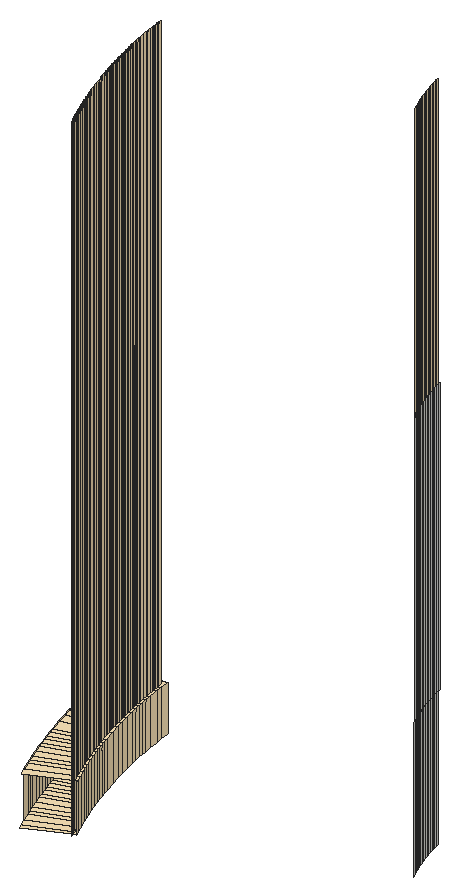
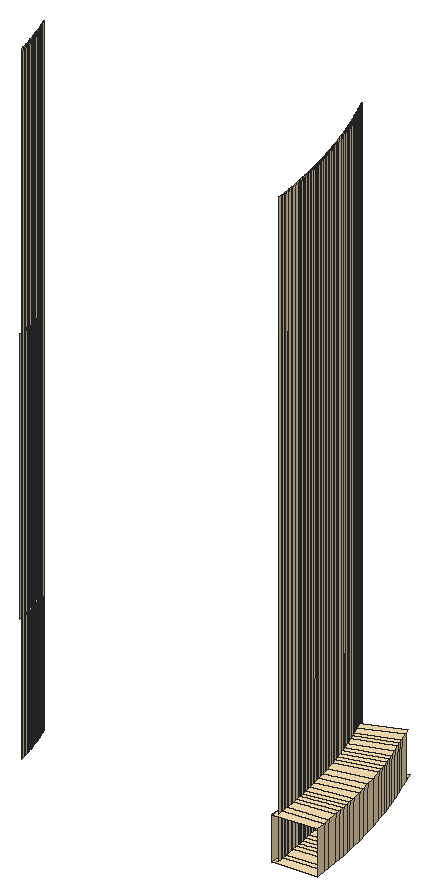
# SketchUp Ruby script. Lengths in inches.
U = 1.inch
M = Sketchup.active_model
def pt(a) = Geom::Point3d.new(a.map { |v| v * U })
def face(e, loops, mat)
  f = e.add_face(loops[0].map { |a| pt(a) })
  loops[1..].each { |l| e.add_face(l.map { |a| pt(a) }).erase! }
  f.material = f.back_material = mat if mat
  f
end
# faces: each face lists its corners as indices into pts; further lists are holes
def faces(e, pts, list, mat = nil) = list.each { |f| face(e, (f[0].is_a?(Array) ? f : [f]).map { |l| l.map { |i| pts[i] } }, mat) }
# xy, xz, yz: faces in a plane at the given z, y or x. An outline is a flat list of corners, or four numbers for a rectangle; further outlines are holes
def ring(l) = l.size == 4 ? [[l[0], l[1]], [l[2], l[1]], [l[2], l[3]], [l[0], l[3]]] : l.each_slice(2).to_a
def flat(e, list, mat, &to3) = list.each { |f| face(e, (f[0].is_a?(Array) ? f : [f]).map { |l| ring(l).map { |u, v| to3.(u, v) } }, mat) }
def xy(e, z, list, mat = nil) = flat(e, list, mat) { |x, y| [x, y, z] }
def xz(e, y, list, mat = nil) = flat(e, list, mat) { |x, z| [x, y, z] }
def yz(e, x, list, mat = nil) = flat(e, list, mat) { |y, z| [x, y, z] }
def lines(e, pts, list) = list.each { |a, b| e.add_line(pt(pts[a]), pt(pts[b])) }
# prism: a flat outline (further loops are holes) pulled along v
def prism(e, loops, v, mat = nil)
  f = face(e, loops, mat); d = Geom::Vector3d.new(v.map { |x| x * U })
  f.pushpull(f.normal.samedirection?(d) ? d.length : -d.length)
end
def box(e, o, s, mat = nil) = prism(e, [[o, [o[0] + s[0], o[1], o[2]], [o[0] + s[0], o[1] + s[1], o[2]], [o[0], o[1] + s[1], o[2]]]], [0, 0, s[2]], mat)
def at(x, y, z, deg = 0) = Geom::Transformation.translation(pt([x, y, z])) * Geom::Transformation.rotation(ORIGIN, Z_AXIS, deg.degrees)
def axes(o, x, y, z) = Geom::Transformation.new([*x, 0, *y, 0, *z, 0, *pt(o).to_a, 1])
def part(name) = M.definitions.add(name)
# library, detail: a bought-in or finely detailed component or shape, given as its bounding box
def library(name, o, s) = part(name).tap { |d| box(d.entities, o, s) }
def detail(e, o, s) = box(e.add_group.entities, o, s)
def put(e, d, t, mat = nil) = e.add_instance(d, t).tap { |i| i.material = mat if mat }
def group(e, t, mat = nil) = e.add_group.tap { |g| g.transformation = t; g.material = mat if mat }.entities
root = M.entities
M.materials.add("1026 AP 7946 SUNNY SIDE UP").color = [254, 231, 186]
xy(root,246,[[6.415,228.386,6.327,228.585,8.035,229.33,8.046,229.304,8.075,229.238,8.09,229.204,8.107,229.167,8.114,229.152],[6.327,228.585,6.202,228.876,7.918,229.598,7.948,229.528,7.974,229.468,7.992,229.428,8.011,229.382,8.035,229.33],[6.202,228.876,6.034,229.281,7.76,229.98,7.779,229.932,7.802,229.878,7.827,229.816,7.853,229.754,7.875,229.7,7.896,229.652,7.918,229.598],[8.114,229.152,8.107,229.167,8.09,229.204,8.075,229.238,8.046,229.304,8.035,229.33,8.16,229.384,8.238,229.208],[6.034,229.281,5.939,229.52,7.672,230.199,7.685,230.165,7.71,230.104,7.738,230.034,7.76,229.98],
  [8.035,229.33,8.011,229.382,7.992,229.428,7.974,229.468,7.948,229.528,7.918,229.598,8.045,229.652,8.16,229.384],[5.939,229.52,5.847,229.76,7.587,230.418,7.594,230.399,7.62,230.333,7.651,230.253,7.669,230.207,7.672,230.199],[7.918,229.598,7.896,229.652,7.875,229.7,7.853,229.754,7.827,229.816,7.802,229.878,7.779,229.932,7.76,229.98,7.888,230.032,8.045,229.652],[5.847,229.76,5.719,230.103,7.467,230.739,7.483,230.693,7.495,230.662,7.505,230.634,7.532,230.5625,7.566,230.473,7.581,230.434,7.587,230.418],[7.76,229.98,7.738,230.034,7.71,230.104,7.685,230.165,7.672,230.199,7.802,230.249,7.888,230.032],
  [5.719,230.103,5.6,230.438,7.355,231.052,7.362,231.03,7.403,230.915,7.411,230.892,7.419,230.87,7.447,230.794,7.467,230.739],[7.672,230.199,7.669,230.207,7.651,230.253,7.62,230.333,7.594,230.399,7.587,230.418,7.718,230.467,7.802,230.249],[7.587,230.418,7.581,230.434,7.566,230.473,7.532,230.5625,7.505,230.634,7.495,230.662,7.483,230.693,7.467,230.739,7.599,230.787,7.718,230.467],[5.6,230.438,5.512,230.696,7.273,231.289,7.277,231.276,7.325,231.137,7.335,231.107,7.355,231.052],[5.512,230.696,5.427,230.953,7.193,231.527,7.249,231.36,7.251,231.352,7.254,231.345,7.273,231.289],
  [7.467,230.739,7.447,230.794,7.419,230.87,7.411,230.892,7.403,230.915,7.362,231.03,7.355,231.052,7.488,231.098,7.599,230.787],[5.427,230.953,5.349,231.195,7.121,231.751,7.175,231.584,7.193,231.527],[7.355,231.052,7.335,231.107,7.325,231.137,7.277,231.276,7.273,231.289,7.407,231.334,7.488,231.098],[5.349,231.195,5.275,231.437,7.051,231.976,7.077,231.893,7.098,231.823,7.101,231.816,7.103,231.808,7.121,231.751],[7.273,231.289,7.254,231.345,7.251,231.352,7.249,231.36,7.193,231.527,7.329,231.571,7.407,231.334],
  [5.275,231.437,5.2,231.686,6.983,232.201,7.001,232.142,7.024,232.063,7.029,232.049,7.033,232.033,7.051,231.976],[7.193,231.527,7.175,231.584,7.121,231.751,7.257,231.794,7.329,231.571],[5.2,231.686,5.053,232.21,6.843,232.694,6.864,232.62,6.884,232.546,6.892,232.517,6.901,232.485,6.931,232.382,6.953,232.304,6.959,232.283,6.966,232.259,6.983,232.201],[7.121,231.751,7.103,231.808,7.101,231.816,7.098,231.823,7.077,231.893,7.051,231.976,7.188,232.018,7.257,231.794],[7.051,231.976,7.033,232.033,7.029,232.049,7.024,232.063,7.001,232.142,6.983,232.201,7.122,232.241,7.188,232.018],
  [6.983,232.201,6.966,232.259,6.959,232.283,6.953,232.304,6.931,232.382,6.901,232.485,6.892,232.517,6.884,232.546,6.864,232.62,6.843,232.694,6.984,232.732,7.122,232.241],[5.053,232.21,4.937,232.658,6.734,233.11,6.738,233.095,6.754,233.031,6.765,232.988,6.778,232.94,6.8,232.857,6.818,232.788,6.828,232.752,6.838,232.713,6.843,232.694],[4.937,232.658,4.845,233.037,6.648,233.46,6.663,233.397,6.679,233.332,6.693,233.275,6.705,233.225,6.719,233.168,6.734,233.11],[6.843,232.694,6.838,232.713,6.828,232.752,6.818,232.788,6.8,232.857,6.778,232.94,6.765,232.988,6.754,233.031,6.738,233.095,6.734,233.11,6.876,233.145,6.984,232.732],[4.845,233.037,4.762,233.401,6.571,233.797,6.578,233.765,6.593,233.701,6.609,233.627,6.623,233.57,6.634,233.52,6.648,233.463,6.648,233.46],
  [6.734,233.11,6.719,233.168,6.705,233.225,6.693,233.275,6.679,233.332,6.663,233.397,6.648,233.46,6.792,233.494,6.876,233.145],[4.762,233.401,4.672,233.828,6.486,234.196,6.489,234.181,6.508,234.087,6.517,234.047,6.524,234.01,6.54,233.94,6.558,233.857,6.568,233.808,6.571,233.797],[6.648,233.46,6.648,233.463,6.634,233.52,6.623,233.57,6.609,233.627,6.593,233.701,6.578,233.765,6.571,233.797,6.716,233.829,6.792,233.494],[6.571,233.797,6.568,233.808,6.558,233.857,6.54,233.94,6.524,234.01,6.517,234.047,6.508,234.087,6.489,234.181,6.486,234.196,6.632,234.226,6.716,233.829],[4.672,233.828,4.61,234.145,6.428,234.489,6.441,234.424,6.461,234.318,6.468,234.286,6.473,234.256,6.486,234.196],
  [4.61,234.145,4.564,234.395,6.385,234.72,6.394,234.67,6.416,234.549,6.421,234.525,6.425,234.503,6.428,234.489],[6.486,234.196,6.473,234.256,6.468,234.286,6.461,234.318,6.441,234.424,6.428,234.489,6.575,234.517,6.632,234.226],[4.564,234.395,4.524,234.629,6.347,234.937,6.349,234.925,6.374,234.781,6.377,234.765,6.379,234.75,6.385,234.72],[6.428,234.489,6.425,234.503,6.421,234.525,6.416,234.549,6.394,234.67,6.385,234.72,6.533,234.747,6.575,234.517],[4.524,234.629,4.48,234.896,6.305,235.185,6.333,235.013,6.335,235.005,6.336,234.998,6.347,234.937],
  [6.385,234.72,6.379,234.75,6.377,234.765,6.374,234.781,6.349,234.925,6.347,234.937,6.496,234.962,6.533,234.747],[4.48,234.896,4.438,235.168,6.267,235.433,6.295,235.246,6.305,235.185],[6.347,234.937,6.336,234.998,6.335,235.005,6.333,235.013,6.305,235.185,6.455,235.208,6.496,234.962],[4.438,235.168,4.369,235.671,6.2,235.908,6.211,235.824,6.222,235.743,6.224,235.728,6.226,235.712,6.247,235.567,6.257,235.494,6.259,235.487,6.26,235.478,6.267,235.433],[6.305,235.185,6.295,235.246,6.267,235.433,6.418,235.455,6.455,235.208],
  [6.267,235.433,6.26,235.478,6.259,235.487,6.257,235.494,6.247,235.567,6.226,235.712,6.224,235.728,6.222,235.743,6.211,235.824,6.2,235.908,6.353,235.928,6.418,235.455],[4.369,235.671,4.333,235.971,6.166,236.179,6.18,236.072,6.189,235.992,6.192,235.97,6.195,235.945,6.2,235.908],[6.2,235.908,6.195,235.945,6.192,235.97,6.189,235.992,6.18,236.072,6.166,236.179,6.32,236.197,6.353,235.928],[4.333,235.971,4.282,236.454,6.117,236.635,6.124,236.5625,6.131,236.491,6.136,236.454,6.14,236.413,6.151,236.318,6.159,236.242,6.163,236.212,6.166,236.179],[6.166,236.179,6.163,236.212,6.159,236.242,6.151,236.318,6.14,236.413,6.136,236.454,6.131,236.491,6.124,236.5625,6.117,236.635,6.272,236.65,6.32,236.197]],"1026 AP 7946 SUNNY SIDE UP")
xy(root,248,[[6.327,228.585,8.16,229.384,8.045,229.652,7.918,229.599,6.202,228.876],[6.202,228.876,7.918,229.599,8.045,229.652,7.888,230.032,7.76,229.98,6.034,229.281],[6.034,229.281,7.76,229.98,7.888,230.032,7.802,230.249,5.939,229.52],[5.939,229.52,7.802,230.249,7.718,230.467,5.847,229.76],[5.847,229.76,7.718,230.467,7.599,230.787,5.72,230.103],
  [5.72,230.103,7.599,230.787,7.488,231.098,5.6,230.438],[5.6,230.438,7.488,231.098,7.407,231.334,5.512,230.696],[5.512,230.696,7.407,231.334,7.329,231.571,5.427,230.953],[5.427,230.953,7.329,231.571,7.258,231.794,5.349,231.195],[5.349,231.195,7.258,231.794,7.189,232.018,5.275,231.437],
  [5.275,231.437,7.189,232.018,7.122,232.242,5.201,231.686],[5.201,231.686,7.122,232.242,6.984,232.732,5.053,232.21],[5.053,232.21,6.984,232.732,6.876,233.145,4.937,232.658],[4.937,232.658,6.876,233.145,6.792,233.494,4.845,233.037],[4.845,233.037,6.792,233.494,6.716,233.829,4.762,233.401],
  [4.762,233.401,6.716,233.829,6.632,234.226,4.672,233.828],[4.672,233.828,6.632,234.226,6.576,234.517,4.61,234.145],[4.61,234.145,6.576,234.517,6.533,234.747,4.565,234.395],[4.565,234.395,6.533,234.747,6.496,234.962,4.524,234.629],[4.524,234.629,6.496,234.962,6.456,235.208,4.48,234.896],
  [4.48,234.896,6.456,235.208,6.418,235.455,4.439,235.168],[4.439,235.168,6.418,235.455,6.353,235.928,4.369,235.671],[4.369,235.671,6.353,235.928,6.32,236.197,6.166,236.179,4.333,235.971],[4.333,235.971,6.166,236.179,6.32,236.197,6.272,236.65,4.282,236.455]],"1026 AP 7946 SUNNY SIDE UP")
p = [[6.202,228.876,246],[6.202,228.876,248],[6.034,229.281,248],[6.034,229.281,246],[8.147,229.079,246],[8.178,229.009,246],
  [8.178,229.009,274],[8.147,229.079,274],[8.107,229.167,246],[8.114,229.152,246],[8.107,229.167,274],[8.046,229.304,246],
  [8.075,229.238,246],[8.075,229.238,274],[8.046,229.304,274],[8.09,229.204,246],[8.09,229.204,274],[8.238,229.208,248],
  [8.238,229.208,246],[8.16,229.384,246],[8.16,229.384,248],[5.939,229.52,248],[5.939,229.52,246],[8.011,229.382,246],
  [8.035,229.33,246],[8.011,229.382,274],[7.974,229.468,246],[7.992,229.428,246],[7.992,229.428,274],[7.974,229.468,274],
  [8.045,229.652,246],[8.045,229.652,248],[5.847,229.76,248],[5.847,229.76,246],[7.918,229.598,246],[7.948,229.528,246],
  [7.948,229.528,274],[7.918,229.598,274],[7.918,229.599,248],[7.896,229.652,246],[7.896,229.652,274],[7.853,229.754,246],
  [7.875,229.7,246],[7.875,229.7,274],[7.853,229.754,274],[7.888,230.032,246],[7.888,230.032,248],[5.72,230.103,248],
  [5.719,230.103,246],[7.802,229.878,246],[7.827,229.816,246],[7.827,229.816,274],[7.802,229.878,274],[7.76,229.98,246],
  [7.779,229.932,246],[7.779,229.932,274],[7.76,229.98,274],[7.76,229.98,248],[7.71,230.104,246],[7.738,230.034,246],
  [7.738,230.034,274],[7.71,230.104,274],[7.802,230.249,246],[7.802,230.249,248],[5.6,230.438,248],[5.6,230.438,246],
  [7.685,230.165,246],[7.685,230.165,274],[7.651,230.253,246],[7.669,230.207,246],[7.669,230.207,274],[7.651,230.253,274],
  [7.672,230.199,246],[7.718,230.467,246],[7.718,230.467,248],[7.594,230.399,246],[7.62,230.333,246],[7.62,230.333,274],
  [7.594,230.399,274],[5.512,230.696,248],[5.512,230.696,246],[7.566,230.473,246],[7.581,230.434,246],[7.581,230.434,274],
  [7.566,230.473,274],[7.587,230.418,246],[7.532,230.5625,246],[7.532,230.5625,274],[7.599,230.787,246],[7.599,230.787,248],
  [7.495,230.662,246],[7.505,230.634,246],[7.505,230.634,274],[7.495,230.662,274],[5.427,230.953,248],[5.427,230.953,246],
  [7.447,230.794,246],[7.467,230.739,246],[7.483,230.693,246],[7.483,230.693,274],[7.447,230.794,274],[7.419,230.87,246],
  [7.419,230.87,274],[7.488,231.098,246],[7.488,231.098,248],[7.362,231.03,246],[7.403,230.915,246],[7.403,230.915,274],
  [7.362,231.03,274],[7.411,230.892,246],[7.411,230.892,274],[5.349,231.195,248],[5.349,231.195,246],[7.335,231.107,246],
  [7.355,231.052,246],[7.335,231.107,274],[7.277,231.276,246],[7.325,231.137,246],[7.325,231.137,274],[7.277,231.276,274],
  [7.33,231.122,246],[7.33,231.122,274],[7.407,231.334,246],[7.407,231.334,248],[5.275,231.437,248],[5.275,231.437,246],
  [7.251,231.352,246],[7.254,231.345,246],[7.254,231.345,274],[7.251,231.352,274],[7.273,231.289,246],[7.329,231.571,246],
  [7.329,231.571,248],[5.201,231.686,248],[5.2,231.686,246],[7.175,231.584,246],[7.193,231.527,246],[7.249,231.36,246],
  [7.249,231.36,274],[7.175,231.584,274],[7.103,231.808,246],[7.121,231.751,246],[7.103,231.808,274],[7.257,231.794,246],
  [7.258,231.794,248],[5.053,232.21,248],[5.053,232.21,246],[7.077,231.893,246],[7.098,231.823,246],[7.098,231.823,274],
  [7.077,231.893,274],[7.101,231.816,246],[7.101,231.816,274],[7.188,232.018,246],[7.189,232.018,248],[7.033,232.033,246],
  [7.051,231.976,246],[7.033,232.033,274],[7.024,232.063,246],[7.029,232.049,246],[7.029,232.049,274],[7.024,232.063,274],
  [7.122,232.241,246],[7.122,232.242,248],[6.966,232.259,246],[6.983,232.201,246],[7.001,232.142,246],[7.001,232.142,274],
  [6.966,232.259,274],[4.937,232.658,248],[4.937,232.658,246],[6.984,232.732,246],[6.984,232.732,248],[6.931,232.382,246],
  [6.953,232.304,246],[6.953,232.304,274],[6.931,232.382,274],[6.959,232.283,246],[6.959,232.283,274],[6.901,232.485,246],
  [6.901,232.485,274],[6.864,232.62,246],[6.884,232.546,246],[6.884,232.546,274],[6.864,232.62,274],[6.892,232.517,246],
  [6.892,232.517,274],[6.838,232.713,246],[6.843,232.694,246],[6.838,232.713,274],[4.845,233.037,248],[4.845,233.037,246],
  [6.828,232.752,246],[6.828,232.752,274],[6.876,233.145,246],[6.876,233.145,248],[6.8,232.857,246],[6.818,232.788,246],
  [6.818,232.788,274],[6.8,232.857,274],[6.765,232.988,246],[6.778,232.94,246],[6.778,232.94,274],[6.765,232.988,274],
  [4.762,233.401,248],[4.762,233.401,246],[6.738,233.095,246],[6.754,233.031,246],[6.754,233.031,274],[6.738,233.095,274],
  [6.719,233.168,246],[6.734,233.11,246],[6.719,233.168,274],[6.792,233.494,246],[6.792,233.494,248],[6.693,233.275,246],
  [6.705,233.225,246],[6.705,233.225,274],[6.693,233.275,274],[6.663,233.397,246],[6.679,233.332,246],[6.679,233.332,274],
  [6.663,233.397,274],[4.672,233.828,248],[4.672,233.828,246],[6.648,233.463,246],[6.648,233.46,246],[6.648,233.463,274],
  [6.623,233.57,246],[6.634,233.52,246],[6.634,233.52,274],[6.623,233.57,274],[6.716,233.829,246],[6.716,233.829,248],
  [6.593,233.701,246],[6.609,233.627,246],[6.609,233.627,274],[6.593,233.701,274],[6.578,233.765,246],[6.578,233.765,274],
  [4.61,234.145,248],[4.61,234.145,246],[6.558,233.857,246],[6.568,233.808,246],[6.568,233.808,274],[6.558,233.857,274],
  [6.571,233.797,246],[6.632,234.226,246],[6.632,234.226,248],[6.524,234.01,246],[6.54,233.94,246],[6.54,233.94,274],
  [6.524,234.01,274],[6.508,234.087,246],[6.517,234.047,246],[6.517,234.047,274],[6.508,234.087,274],[4.565,234.395,248],
  [4.564,234.395,246],[6.489,234.181,246],[6.489,234.181,274],[19.037,234.119,252],[18.975,234.263,252],[18.975,234.263,246],
  [19.037,234.119,246],[6.473,234.256,246],[6.486,234.196,246],[6.473,234.256,274],[6.575,234.517,246],[6.576,234.517,248],
  [18.987,234.234,246],[18.9375,234.35,246],[18.9375,234.35,276],[18.987,234.234,276],[6.441,234.424,246],[6.461,234.318,246],
  [6.461,234.318,274],[6.441,234.424,274],[6.468,234.286,246],[6.468,234.286,274],[18.89,234.466,246],[18.89,234.466,276],
  [18.913,234.408,252],[18.913,234.408,246],[4.524,234.629,248],[4.524,234.629,246],[6.425,234.503,246],[6.428,234.489,246],
  [6.425,234.503,274],[18.854,234.553,252],[18.854,234.553,246],[6.394,234.67,246],[6.416,234.549,246],[6.416,234.549,274],
  [6.394,234.67,274],[6.421,234.525,246],[6.421,234.525,274],[6.533,234.747,246],[6.533,234.747,248],[18.843,234.583,246],
  [18.843,234.583,276],[4.48,234.896,248],[4.48,234.896,246],[18.797,234.7,246],[18.797,234.7,276],[18.797,234.7,252],
  [18.797,234.7,246],[6.377,234.765,246],[6.379,234.75,246],[6.379,234.75,274],[6.377,234.765,274],[6.385,234.72,246],
  [6.496,234.962,246],[6.496,234.962,248],[18.742,234.847,252],[18.742,234.847,246],[18.753,234.817,246],[18.753,234.817,276],
  [6.349,234.925,246],[6.374,234.781,246],[6.374,234.781,274],[6.349,234.925,274],[18.709,234.935,246],[18.709,234.935,276],
  [18.688,234.994,252],[18.688,234.994,246],[4.439,235.168,248],[4.438,235.168,246],[6.336,234.998,246],[6.347,234.937,246],
  [6.336,234.998,274],[18.667,235.054,246],[18.667,235.054,276],[6.295,235.246,246],[6.305,235.185,246],[6.333,235.013,246],
  [6.333,235.013,274],[6.295,235.246,274],[6.335,235.005,246],[6.335,235.005,274],[6.455,235.208,246],[6.456,235.208,248],
  [18.637,235.143,252],[18.637,235.143,246],[18.627,235.172,246],[18.627,235.172,276],[18.587,235.292,252],[18.587,235.292,246],
  [4.369,235.671,248],[4.369,235.671,246],[6.26,235.478,246],[6.267,235.433,246],[6.26,235.478,274],[6.418,235.455,246],
  [6.418,235.455,248],[18.587,235.292,246],[18.587,235.292,276],[18.549,235.412,246],[18.549,235.412,276],[18.54,235.442,252],
  [18.54,235.442,246],[18.512,235.532,246],[18.512,235.532,276],[18.494,235.592,252],[18.494,235.592,246],[6.247,235.567,246],
  [6.257,235.494,246],[6.257,235.494,274],[6.247,235.567,274],[6.259,235.487,246],[6.259,235.487,274],[6.353,235.928,246],
  [6.353,235.928,248],[18.476,235.652,246],[18.476,235.652,276],[6.226,235.712,246],[6.226,235.712,274],[18.451,235.743,252],
  [18.451,235.743,246],[4.333,235.971,248],[4.333,235.971,246],[6.211,235.824,246],[6.222,235.743,246],[6.222,235.743,274],
  [6.211,235.824,274],[6.224,235.728,246],[6.224,235.728,274],[18.442,235.773,246],[18.442,235.773,276],[18.409,235.894,252],
  [18.409,235.894,246],[6.195,235.945,246],[6.2,235.908,246],[6.195,235.945,274],[18.409,235.894,246],[18.409,235.894,276],
  [6.192,235.97,246],[6.192,235.97,274],[6.32,236.197,246],[6.32,236.197,248],[18.377,236.016,246],[18.377,236.016,276],
  [18.369,236.046,252],[18.369,236.046,246],[4.282,236.455,248],[4.282,236.454,246],[6.18,236.072,246],[6.189,235.992,246],
  [6.189,235.992,274],[6.18,236.072,274],[18.346,236.138,246],[18.346,236.138,276],[18.332,236.199,252],[18.332,236.199,246],
  [6.166,236.179,246],[6.166,236.179,274],[6.166,236.179,248],[18.317,236.26,246],[18.317,236.26,276],[6.151,236.318,246],
  [6.159,236.242,246],[6.159,236.242,274],[6.151,236.318,274],[6.163,236.212,246],[6.163,236.212,274],[6.272,236.65,246],
  [6.272,236.65,248],[18.296,236.352,252],[18.296,236.352,246],[6.14,236.413,246],[6.14,236.413,274],[18.289,236.382,246],
  [18.289,236.382,276],[18.975,234.263,264],[18.913,234.408,264],[18.913,234.408,252],[18.975,234.263,252],[18.854,234.553,264],
  [18.854,234.553,252],[18.797,234.7,264],[18.797,234.7,252],[18.742,234.847,264],[18.742,234.847,252],[18.688,234.994,264],
  [18.688,234.994,252],[18.637,235.143,264],[18.637,235.143,252],[18.587,235.292,264],[18.587,235.292,252],[18.54,235.442,264],
  [18.54,235.442,252],[18.494,235.592,264],[18.494,235.592,252],[18.451,235.743,264],[18.451,235.743,252],[18.409,235.894,264],
  [18.409,235.894,252],[18.369,236.046,264],[18.369,236.046,252],[18.332,236.199,264],[18.332,236.199,252],[18.296,236.352,264],
  [18.296,236.352,252],[18.262,236.505,264],[18.262,236.505,252]]
faces(root,p,[[0,1,2,3],[4,5,6,7],[8,9,4,7,10],[11,12,13,14],[12,15,16,13],[15,8,10,16],[17,18,19,20],[3,2,21,22],
  [23,24,11,14,25],[26,27,28,29],[27,23,25,28],[20,19,30,31],[22,21,32,33],[34,35,36,37,38],[35,26,29,36],[39,34,38,37,40],
  [41,42,43,44],[42,39,40,43],[31,30,45,46],[33,32,47,48],[49,50,51,52],[50,41,44,51],[53,54,55,56,57],[54,49,52,55],
  [58,59,60,61],[59,53,57,56,60],[46,45,62,63],[48,47,64,65],[66,58,61,67],[68,69,70,71],[69,72,66,67,70],[63,62,73,74],
  [75,76,77,78],[76,68,71,77],[65,64,79,80],[81,82,83,84],[82,85,75,78,83],[86,81,84,87],[74,73,88,89],[90,91,92,93],
  [91,86,87,92],[80,79,94,95],[96,97,98,99,100],[98,90,93,99],[101,96,100,102],[89,88,103,104],[105,106,107,108],[106,109,110,107],
  [109,101,102,110],[95,94,111,112],[113,114,105,108,115],[116,117,118,119],[117,120,121,118],[120,113,115,121],[104,103,122,123],[112,111,124,125],
  [126,127,128,129],[127,130,116,119,128],[123,122,131,132],[125,124,133,134],[135,136,137,138,139],[137,126,129,138],[140,141,135,139,142],[132,131,143,144],
  [134,133,145,146],[147,148,149,150],[148,151,152,149],[151,140,142,152],[144,143,153,154],[155,156,147,150,157],[158,159,160,161],[159,155,157,160],
  [154,153,162,163],[164,165,166,167,168],[166,158,161,167],[146,145,169,170],[163,162,171,172],[173,174,175,176],[174,177,178,175],[177,164,168,178],
  [179,173,176,180],[181,182,183,184],[182,185,186,183],[185,179,180,186],[187,188,181,184,189],[170,169,190,191],[192,187,189,193],[172,171,194,195],
  [196,197,198,199],[197,192,193,198],[200,201,202,203],[201,196,199,202],[191,190,204,205],[206,207,208,209],[207,200,203,208],[210,211,206,209,212],
  [195,194,213,214],[215,216,217,218],[216,210,212,217],[219,220,221,222],[220,215,218,221],[205,204,223,224],[225,226,219,222,227],[228,229,230,231],
  [229,225,227,230],[214,213,232,233],[234,235,236,237],[235,228,231,236],[238,234,237,239],[224,223,240,241],[242,243,244,245],[243,246,238,239,244],
  [233,232,247,248],[249,250,251,252],[250,242,245,251],[253,254,255,256],[254,249,252,255],[241,240,257,258],[259,253,256,260],[265,266,259,260,267],
  [248,247,268,269],[270,271,272,273],[274,275,276,277],[275,278,279,276],[278,265,267,279],[271,280,281,272],[258,257,284,285],[286,287,274,277,288],
  [291,292,293,294],[292,295,296,293],[295,286,288,296],[269,268,297,298],[280,299,300,281],[285,284,301,302],[299,303,304,300],[307,308,309,310],
  [308,311,291,294,309],[298,297,312,313],[303,316,317,304],[318,319,320,321],[319,307,310,320],[316,322,323,317],[302,301,326,327],[328,329,318,321,330],
  [322,331,332,323],[333,334,335,336,337],[335,338,339,336],[338,328,330,339],[313,312,340,341],[331,344,345,332],[327,326,348,349],[350,351,333,337,352],
  [341,340,353,354],[344,355,356,345],[355,357,358,356],[357,361,362,358],[365,366,367,368],[366,369,370,367],[369,350,352,370],[354,353,371,372],
  [361,373,374,362],[375,365,368,376],[349,348,379,380],[381,382,383,384],[382,385,386,383],[385,375,376,386],[373,387,388,374],[391,392,381,384,393],
  [387,394,395,388],[396,391,393,397],[372,371,398,399],[394,400,401,395],[380,379,404,405],[406,407,408,409],[407,396,397,408],[400,410,411,401],
  [414,406,409,415,416],[410,417,418,411],[419,420,421,422],[420,423,424,421],[423,414,416,415,424],[399,398,425,426],[429,419,422,430],[417,431,432,418]],"1026 AP 7946 SUNNY SIDE UP")
faces(root,p,[[261,262,263,264],[262,282,283,263],[282,289,290,283],[289,305,306,290],[305,314,315,306],[314,324,325,315],[324,342,343,325],[342,346,347,343],
  [346,359,360,347],[359,363,364,360],[363,377,378,364],[377,389,390,378],[389,402,403,390],[402,412,413,403],[412,427,428,413],[433,434,435,436],
  [434,437,438,435],[437,439,440,438],[439,441,442,440],[441,443,444,442],[443,445,446,444],[445,447,448,446],[447,449,450,448],[449,451,452,450],
  [451,453,454,452],[453,455,456,454],[455,457,458,456],[457,459,460,458],[459,461,462,460],[461,463,464,462]])
